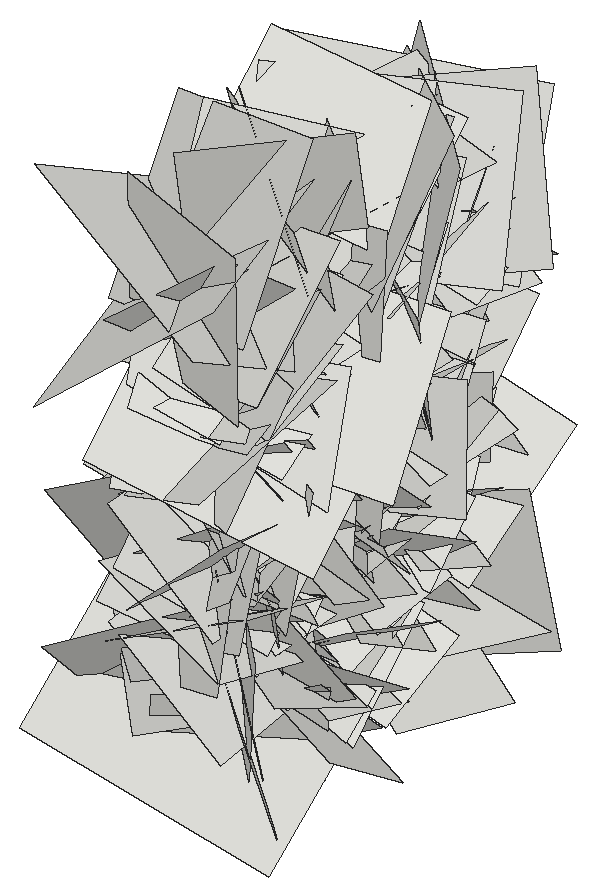
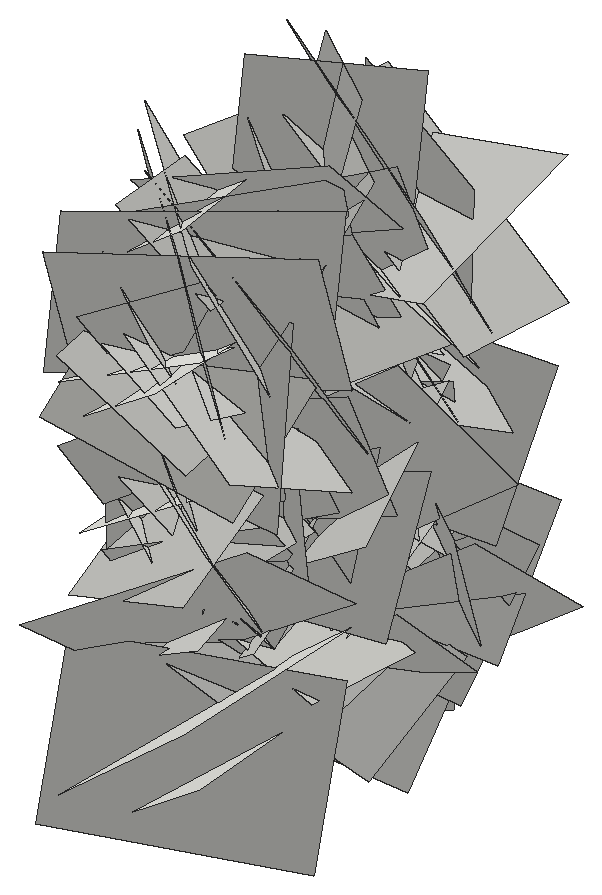
# SketchUp Ruby script. Lengths in inches.
U = 1.inch
M = Sketchup.active_model
def pt(a) = Geom::Point3d.new(a.map { |v| v * U })
def face(e, loops, mat)
  f = e.add_face(loops[0].map { |a| pt(a) })
  loops[1..].each { |l| e.add_face(l.map { |a| pt(a) }).erase! }
  f.material = f.back_material = mat if mat
  f
end
# faces: each face lists its corners as indices into pts; further lists are holes
def faces(e, pts, list, mat = nil) = list.each { |f| face(e, (f[0].is_a?(Array) ? f : [f]).map { |l| l.map { |i| pts[i] } }, mat) }
# xy, xz, yz: faces in a plane at the given z, y or x. An outline is a flat list of corners, or four numbers for a rectangle; further outlines are holes
def ring(l) = l.size == 4 ? [[l[0], l[1]], [l[2], l[1]], [l[2], l[3]], [l[0], l[3]]] : l.each_slice(2).to_a
def flat(e, list, mat, &to3) = list.each { |f| face(e, (f[0].is_a?(Array) ? f : [f]).map { |l| ring(l).map { |u, v| to3.(u, v) } }, mat) }
def xy(e, z, list, mat = nil) = flat(e, list, mat) { |x, y| [x, y, z] }
def xz(e, y, list, mat = nil) = flat(e, list, mat) { |x, z| [x, y, z] }
def yz(e, x, list, mat = nil) = flat(e, list, mat) { |y, z| [x, y, z] }
def lines(e, pts, list) = list.each { |a, b| e.add_line(pt(pts[a]), pt(pts[b])) }
# prism: a flat outline (further loops are holes) pulled along v
def prism(e, loops, v, mat = nil)
  f = face(e, loops, mat); d = Geom::Vector3d.new(v.map { |x| x * U })
  f.pushpull(f.normal.samedirection?(d) ? d.length : -d.length)
end
def box(e, o, s, mat = nil) = prism(e, [[o, [o[0] + s[0], o[1], o[2]], [o[0] + s[0], o[1] + s[1], o[2]], [o[0], o[1] + s[1], o[2]]]], [0, 0, s[2]], mat)
def at(x, y, z, deg = 0) = Geom::Transformation.translation(pt([x, y, z])) * Geom::Transformation.rotation(ORIGIN, Z_AXIS, deg.degrees)
def axes(o, x, y, z) = Geom::Transformation.new([*x, 0, *y, 0, *z, 0, *pt(o).to_a, 1])
def part(name) = M.definitions.add(name)
# library, detail: a bought-in or finely detailed component or shape, given as its bounding box
def library(name, o, s) = part(name).tap { |d| box(d.entities, o, s) }
def detail(e, o, s) = box(e.add_group.entities, o, s)
def put(e, d, t, mat = nil) = e.add_instance(d, t).tap { |i| i.material = mat if mat }
def group(e, t, mat = nil) = e.add_group.tap { |g| g.transformation = t; g.material = mat if mat }.entities
root = M.entities
c1 = part("Component\#6")
p = [[0.01,0,0],[0,3.24,4.54],[4.32,3.24,4.54],[4.33,0,0]]
faces(c1.entities,p,[[0,1,2,3]])
put(root,c1,axes([18.5,163.2,33.68],[-0.16473,-1.2102,0.57798],[-0.2383,0.59712,1.18983],[-1.40149,0.04071,-0.27024]))
put(root,c1,axes([18.5,157.9,37.93],[-0.24747,1.3445,0.30187],[0.11522,0.32319,-1.35538],[-1.4561,-0.20293,-0.15855]))
put(root,c1,axes([18.5,168.45,29.92],[-0.2904,-0.81126,-1.09363],[0.15157,-1.12651,0.79984],[-1.4354,0.04517,0.30571]))
put(root,c1,axes([18.5,159.18,36.25],[-0.04304,0.74935,1.15311],[-0.14712,1.14549,-0.74928],[-1.45028,-0.13844,0.04179]))
put(root,c1,axes([18.5,165.11,34.6875],[-0.03998,0.77126,1.05992],[-0.2457,1.03973,-0.76482],[-1.36759,-0.20934,0.10642]))
put(root,c1,axes([18.5,172.42,21.79],[-0.22827,-1.35966,0.24048],[0.1567,0.21929,1.3722],[-1.45519,0.2369,0.11004]))
put(root,c1,axes([18.5,158.06,26.05],[-0.19995,0.52409,1.06255],[-0.00833,1.07535,-0.5318],[-1.25583,-0.09057,-0.16565]))
put(root,c1,axes([18.5,166.62,31.96],[-0.21061,0.75098,-0.921],[0.02022,-0.93165,-0.76377],[-1.25951,-0.14053,0.14175]))
put(root,c1,axes([18.5,158.99,33.95],[-0.09747,0.08794,1.12692],[-0.17247,1.11783,-0.1005],[-1.18568,-0.16983,-0.07802]))
put(root,c1,axes([18.5,173.53,27.66],[-0.08068,-0.97468,-0.75893],[-0.01331,-0.75972,0.97695],[-1.30935,0.06778,0.03684]))
put(root,c1,axes([18.5,171.44,26.6],[0.03428,0.27698,-1.26013],[-0.06702,-1.25867,-0.27828],[-1.36598,0.0687,-0.01797]))
put(root,c1,axes([18.5,172.54,38.57],[0.12011,-0.4932,-1.18141],[-0.20578,-1.17893,0.47355],[-1.34134,0.1367,-0.17844]))
put(root,c1,axes([18.5,160.96,32.62],[-0.12215,0.75895,-0.88724],[-0.014,-0.89234,-0.7616],[-1.23753,-0.06482,0.09619]))
put(root,c1,axes([18.5,164.92,23.28],[-0.02573,-1.02703,-0.88101],[0.12942,-0.87922,1.02158],[-1.42847,-0.06116,0.10843]))
put(root,c1,axes([18.5,165.55,34.43],[0.04885,1.13911,0.54464],[-0.08516,0.54654,-1.13629],[-1.33566,0.00681,0.09237]))
put(root,c1,axes([18.5,166.97,25.06],[0.03339,-0.82276,-0.77538],[-0.30966,-0.75526,0.78954],[-1.15769,0.17829,-0.23355]))
put(root,c1,axes([18.5,159.8,34.2],[0.03301,0.77795,0.85676],[-0.24326,0.8442,-0.75821],[-1.20233,-0.14944,0.17692]))
put(root,c1,axes([18.5,169.63,32.59],[-0.01533,-0.4611,-1.03377],[-0.17767,-1.02158,0.45801],[-1.18663,0.15892,-0.05522]))
put(root,c1,axes([18.5,160.22,28.4],[-0.15479,0.80897,-0.76348],[0.02106,-0.76802,-0.81757],[-1.17891,-0.11994,0.08565]))
put(root,c1,axes([18.5,163.85,26.9],[-0.03329,1.04875,0.11229],[-0.24045,0.10299,-1.02538],[-1.09187,-0.05466,0.22238]))
put(root,c1,axes([18.5,168.84,39.14],[-0.0295,-0.69575,-0.73723],[-0.22295,-0.71749,0.68506],[-1.05113,0.17171,-0.12461]))
put(root,c1,axes([18.5,167.41,29.34],[0.20833,-0.42173,1.22713],[-0.0869,1.23461,0.43743],[-1.37269,-0.14217,0.15855]))
put(root,c1,axes([18.5,163.625,35.04],[-0.27654,-0.44632,0.88094],[0.09901,0.89592,0.48157],[-1.04211,0.20356,-0.18801]))
put(root,c1,axes([14.53,163.13,28.77],[-0.13219,-0.55975,0.33448],[-0.05965,0.34851,0.56225],[0.68862,-0.07726,0.11291]))
put(root,c1,axes([18.5,171.44,27.64],[-0.05126,-0.8571,0.56567],[-0.11133,0.56746,0.85083],[-1.08285,-0.01777,-0.11425]))
put(root,c1,axes([18.5,167.53,29.6],[-0.04916,0.6172,0.8297],[-0.08211,0.82613,-0.61887],[-1.09305,-0.08981,0.00917]))
put(root,c1,axes([18.5,170.89,20.28],[-0.12274,-1.02279,0.17958],[0.0333,0.17716,1.02926],[-1.10024,0.11946,0.01112]))
put(root,c1,axes([18.5,169.04,36.23],[0.04162,0.78981,-0.64322],[-0.24351,-0.62024,-0.77563],[-1.05189,0.17484,0.15411]))
put(root,c1,axes([14.53,163.1,21.29],[-0.03251,-0.459,0.52355],[-0.17075,0.51451,0.44164],[0.71801,0.10157,0.12873]))
put(root,c1,axes([18.5,158.58,28.72],[-0.17742,0.80309,0.64454],[0.10421,0.66248,-0.79991],[-1.08655,-0.0676,-0.18196]))
put(root,c1,axes([18.5,168.75,37.98],[0.06882,-0.53698,-1.12739],[0.1022,-1.12338,0.54063],[-1.31971,-0.115,-0.01692]))
put(root,c1,axes([18.5,166.67,25.47],[0.29316,-1.18227,0.54308],[-0.10516,0.53443,1.21398],[-1.37509,-0.29293,0.02294]))
put(root,c1,axes([14.53,169.1,21.1],[-0.05323,-0.42134,0.48328],[-0.06346,0.48572,0.41725],[0.67666,0.01241,0.07715]))
put(root,c1,axes([18.5,166.55,31.56],[-0.0814,0.41102,-0.8284],[-0.17089,-0.82447,-0.39413],[-0.96524,0.11131,0.13964]))
put(root,c1,axes([14.53,165.91,24.52],[0.03596,-0.58924,0.24858],[-0.15481,0.23521,0.57749],[0.65999,0.08727,0.12191]))
put(root,c1,axes([18.5,159.57,38.3125],[0.19748,1.37219,0.09956],[0.15298,0.08042,-1.37849],[-1.4503,0.19533,-0.13185]))
put(root,c1,axes([18.5,160.7,27.63],[0.09928,0.64406,-0.88513],[-0.13228,-0.87629,-0.65083],[-1.15276,0.15602,-0.00154]))
put(root,c1,axes([14.53,161.42,33.85],[-0.12931,-0.58697,0.4315],[-0.06321,0.44408,0.58723],[0.76963,-0.06214,0.12073]))
put(root,c1,axes([18.5,164.67,22.86],[0.07455,-1.03669,0.46758],[-0.01691,0.46753,1.03897],[-1.20537,-0.07068,0.01434]))
put(root,c1,axes([18.5,169.13,31.47],[-0.22896,-0.22184,-0.76377],[-0.12794,-0.77313,0.25869],[-0.83329,0.17965,0.17014]))
put(root,c1,axes([14.53,168.14,25.37],[-0.00005,-0.54267,0.44601],[-0.16088,0.43548,0.52984],[0.72699,0.09633,0.11728]))
put(root,c1,axes([14.53,167.47,38.84],[-0.19203,-0.25676,-0.78485],[-0.09527,-0.79261,0.28005],[0.87013,-0.14344,-0.14255]))
put(root,c1,axes([18.5,162.55,24.47],[-0.08094,0.6993,-0.63815],[-0.06519,-0.64254,-0.69674],[-1.00139,-0.01469,0.09694]))
put(root,c1,axes([18.5,168.37,37.02],[0.06582,-0.55881,-0.84289],[-0.17414,-0.83883,0.54402],[-1.05774,0.10333,-0.14201]))
put(root,c1,axes([14.53,168.24,29.62],[-0.00844,-0.1319,-0.59476],[-0.00779,-0.59475,0.132],[0.64572,-0.0089,-0.00618]))
put(root,c1,axes([14.53,163.79,31.02],[-0.0186,-0.39942,0.51021],[-0.04828,0.50989,0.39761],[0.68514,0.02509,0.04187]))
put(root,c1,axes([14.53,167.3,30.05],[-0.09755,-0.36279,0.79394],[-0.2327,0.7823,0.33203],[0.89554,0.16375,0.17276]))
put(root,c1,axes([14.53,166.74,28.03],[-0.20581,0.5378,0.53941],[0.0447,0.5634,-0.54654],[0.80617,0.10606,0.16802]))
put(root,c1,axes([14.53,165.16,26.22],[0.00662,-0.41647,0.48084],[-0.04981,0.47925,0.41571],[0.67246,0.0396,0.02606]))
put(root,c1,axes([18.5,162.15,25.43],[0.09766,0.84172,-0.54191],[-0.18116,-0.52299,-0.84139],[-1.04557,0.16923,0.09516]))
put(root,c1,axes([14.53,170.38,37.22],[-0.01844,-0.65259,0.06973],[-0.0154,0.07012,0.65262],[0.69551,-0.01575,0.0163]))
put(root,c1,axes([18.5,159.15,32.85],[0.28722,0.93511,0.86971],[0.00467,0.88838,-0.95656],[-1.35365,0.20148,0.18123]))
put(root,c1,axes([14.53,158.35,30.49],[-0.08461,0.81055,-0.03501],[-0.12527,-0.04642,-0.80528],[0.85081,0.07377,-0.12204]))
put(root,c1,axes([14.53,168.23,31.98],[-0.11552,-0.73847,0.10601],[0.00435,0.10653,0.74638],[0.79079,-0.10846,0.01138]))
put(root,c1,axes([14.53,162.33,29.83],[-0.22776,0.38392,-0.75072],[0.01782,-0.77261,-0.39993],[0.89361,0.11326,-0.18337]))
put(root,c1,axes([18.5,165.04,27.71],[0.04822,0.07219,0.94774],[-0.14201,0.93984,-0.06516],[-0.99746,-0.13032,0.05509]))
put(root,c1,axes([14.53,171.91,32.4],[0.07209,-0.36069,-0.54144],[-0.07785,-0.54516,0.35394],[0.6852,-0.024,0.09718]))
put(root,c1,axes([18.5,167.29,35.58],[-0.17595,-0.29467,-0.74084],[-0.05215,-0.7515,0.30993],[-0.84352,0.10793,0.13537]))
put(root,c1,axes([18.5,157.3125,32.29],[0.25179,1.05256,0.51222],[-0.06429,0.53303,-1.06718],[-1.23914,0.18623,0.15945]))
put(root,c1,axes([14.53,168.82,35.84],[0.04533,0.37689,0.51175],[-0.01637,0.51337,-0.3768],[0.67349,-0.01289,-0.04361]))
put(root,c1,axes([14.53,159.46,22.85],[-0.09982,-0.0635,0.89488],[-0.1784,0.88507,0.04509],[0.93408,0.16225,0.10424]))
put(root,c1,axes([14.53,160.06,22.6],[-0.02839,-0.24478,0.77995],[-0.15528,0.76918,0.23637],[0.85248,0.13195,0.06903]))
put(root,c1,axes([14.53,159.67,28.14],[-0.12868,0.67272,0.52517],[-0.08613,0.51893,-0.68352],[0.90053,0.14576,0.00967]))
put(root,c1,axes([14.53,158.39,26.84],[-0.02686,0.84806,0.10272],[-0.17857,0.09579,-0.83237],[0.88773,0.04493,-0.16432]))
put(root,c1,axes([14.53,169.17,27.35],[0.00515,-0.4485,-0.48712],[0.04455,-0.48594,0.44784],[0.70046,0.0342,-0.02491]))
put(root,c1,axes([18.5,161.79,25.53],[-0.01152,-0.82607,0.19056],[-0.15176,0.18963,0.81386],[-0.88572,-0.02175,-0.14193]))
put(root,c1,axes([18.5,164.2,31.01],[0.06613,-0.18181,-0.96198],[-0.02897,-0.96387,0.1804],[-1.03734,0.01533,-0.06637]))
put(root,c1,axes([14.53,169.92,30.86],[0.08798,0.07784,-0.70174],[-0.08853,-0.70052,-0.08758],[0.74315,-0.09267,0.07264]))
put(root,c1,axes([18.5,162.32,28.44],[-0.12821,-0.42216,-0.69512],[0.01339,-0.70366,0.42514],[-0.86197,0.05186,0.11]))
put(root,c1,axes([18.5,166.33,22.3],[0.05809,-0.87115,0.26873],[-0.09257,0.26296,0.87026],[-0.96191,-0.07791,-0.06752]))
put(root,c1,axes([18.5,171.77,39.47],[0.25632,-0.1505,-1.28885],[0.2021,-1.29268,0.18672],[-1.36053,-0.22038,-0.21508]))
put(root,c1,axes([14.53,167.69,34.89],[0.01272,-0.59445,-0.3878],[0.01652,-0.38754,0.59453],[0.75216,0.01856,-0.0065]))
put(root,c1,axes([14.53,168.18,25.35],[0.0356,-0.79141,-0.13903],[-0.13499,-0.14264,0.78117],[0.84098,0.01061,0.13127]))
put(root,c1,axes([18.5,163.85,33.45],[0.03445,-0.73428,-0.4148],[-0.17499,-0.41262,0.71747],[-0.87664,0.05351,-0.15952]))
put(root,c1,axes([18.5,158.45,30.92],[0.16236,0.46297,0.88251],[-0.09478,0.89566,-0.45434],[-1.05211,-0.00924,0.17712]))
put(root,c1,axes([18.5,166.53,31.68],[0.02185,0.89564,-0.0065],[-0.05171,-0.00537,-0.89456],[-0.948,0.02094,0.04865]))
put(root,c1,axes([18.5,171.21,38.93],[0.24063,-0.51313,-1.11059],[0.16085,-1.10901,0.54342],[-1.28679,-0.23458,-0.13976]))
put(root,c1,axes([14.53,171.89,34.33],[-0.10287,-0.74562,-0.1631],[0.15609,-0.17961,0.73351],[0.79385,-0.06131,-0.16536]))
put(root,c1,axes([18.5,162.43,26.35],[-0.02315,-0.70596,0.51236],[0.01203,0.51225,0.70629],[-0.92456,0.02434,-0.00364]))
put(root,c1,axes([18.5,162.61,28.57],[0.04222,-0.49534,0.62953],[-0.20196,0.60636,0.48917],[-0.82474,-0.17384,-0.08755]))
put(root,c1,axes([18.5,162.92,24.26],[-0.16568,0.16434,-0.80239],[0.1251,-0.80382,-0.18763],[-0.85913,-0.14874,0.12742]))
put(root,c1,axes([18.5,164.5,23.79],[-0.04443,0.667,0.37408],[-0.11412,0.36576,-0.66423],[-0.80255,-0.08894,0.07374]))
put(root,c1,axes([18.5,168.875,35.8],[-0.07444,0.7996,-0.0855],[-0.00091,-0.0859,-0.80263],[-0.85241,-0.06974,0.00832]))
put(root,c1,axes([14.53,164.96,33.58],[0.03363,-0.67551,-0.53197],[-0.14584,-0.52946,0.66412],[0.89967,-0.06058,0.12754]))
put(root,c1,axes([14.53,169.82,24.93],[0.00586,-0.68753,0.27068],[0.05817,0.27032,0.6855],[0.78107,-0.01497,-0.05308]))
put(root,c1,axes([18.5,164.8,26.41],[-0.06555,-0.88967,-0.10275],[0.1194,-0.1099,0.88381],[-0.94178,0.04799,0.1192]))
put(root,c1,axes([18.5,163.99,40.83],[-0.08038,0.23372,-0.81219],[0.10222,-0.80774,-0.24144],[-0.89001,-0.11388,0.04562]))
put(root,c1,axes([18.5,167.51,23.32],[0.04127,-0.8056,0.43064],[0.05085,0.43224,0.80425],[-0.96695,-0.01165,0.06068]))
put(root,c1,axes([18.5,164.95,29.96],[0.04265,0.57286,-0.52342],[-0.15347,-0.50938,-0.56862],[-0.80809,0.12697,0.08036]))
put(root,c1,axes([14.53,164.95,29.96],[-0.04265,0.57286,-0.52342],[0.15347,-0.50938,-0.56862],[0.80809,0.12697,0.08036]))
put(root,c1,axes([14.53,167.51,23.32],[-0.04127,-0.8056,0.43064],[-0.05085,0.43224,0.80425],[0.96695,-0.01165,0.06068]))
put(root,c1,axes([14.53,163.99,40.83],[0.08038,0.23372,-0.81219],[-0.10222,-0.80774,-0.24144],[0.89001,-0.11388,0.04562]))
put(root,c1,axes([14.53,164.8,26.41],[0.06555,-0.88967,-0.10275],[-0.1194,-0.1099,0.88381],[0.94178,0.04799,0.1192]))
put(root,c1,axes([18.5,169.82,24.93],[-0.00586,-0.68753,0.27068],[-0.05817,0.27032,0.6855],[-0.78107,-0.01497,-0.05308]))
put(root,c1,axes([18.5,164.96,33.58],[-0.03363,-0.67551,-0.53197],[0.14584,-0.52946,0.66412],[-0.89967,-0.06058,0.12754]))
put(root,c1,axes([14.53,168.875,35.8],[0.07444,0.7996,-0.0855],[0.00091,-0.0859,-0.80263],[0.85241,-0.06974,0.00832]))
put(root,c1,axes([14.53,164.5,23.79],[0.04443,0.667,0.37408],[0.11412,0.36576,-0.66423],[0.80255,-0.08894,0.07374]))
put(root,c1,axes([14.53,162.92,24.26],[0.16568,0.16434,-0.80239],[-0.1251,-0.80382,-0.18763],[0.85913,-0.14874,0.12742]))
put(root,c1,axes([14.53,162.61,28.57],[-0.04222,-0.49534,0.62953],[0.20196,0.60636,0.48917],[0.82474,-0.17384,-0.08755]))
put(root,c1,axes([14.53,162.43,26.35],[0.02315,-0.70596,0.51236],[-0.01203,0.51225,0.70629],[0.92456,0.02434,-0.00364]))
put(root,c1,axes([18.5,171.89,34.33],[0.10287,-0.74562,-0.1631],[-0.15609,-0.17961,0.73351],[-0.79385,-0.06131,-0.16536]))
put(root,c1,axes([14.53,171.21,38.93],[-0.24063,-0.51313,-1.11059],[-0.16085,-1.10901,0.54342],[1.28679,-0.23458,-0.13976]))
put(root,c1,axes([14.53,166.53,31.68],[-0.02185,0.89564,-0.0065],[0.05171,-0.00537,-0.89456],[0.948,0.02094,0.04865]))
put(root,c1,axes([14.53,158.45,30.92],[-0.16236,0.46297,0.88251],[0.09478,0.89566,-0.45434],[1.05211,-0.00924,0.17712]))
put(root,c1,axes([14.53,163.85,33.45],[-0.03445,-0.73428,-0.4148],[0.17499,-0.41262,0.71747],[0.87664,0.05351,-0.15952]))
put(root,c1,axes([18.5,168.18,25.35],[-0.0356,-0.79141,-0.13903],[0.13499,-0.14264,0.78117],[-0.84098,0.01061,0.13127]))
put(root,c1,axes([18.5,167.69,34.89],[-0.01272,-0.59445,-0.3878],[-0.01652,-0.38754,0.59453],[-0.75216,0.01856,-0.0065]))
put(root,c1,axes([14.53,171.77,39.47],[-0.25632,-0.1505,-1.28885],[-0.2021,-1.29268,0.18672],[1.36053,-0.22038,-0.21508]))
put(root,c1,axes([14.53,166.33,22.3],[-0.05809,-0.87115,0.26873],[0.09257,0.26296,0.87026],[0.96191,-0.07791,-0.06752]))
put(root,c1,axes([14.53,162.32,28.44],[0.12821,-0.42216,-0.69512],[-0.01339,-0.70366,0.42514],[0.86197,0.05186,0.11]))
put(root,c1,axes([18.5,169.92,30.86],[-0.08798,0.07784,-0.70174],[0.08853,-0.70052,-0.08758],[-0.74315,-0.09267,0.07264]))
put(root,c1,axes([14.53,164.2,31.01],[-0.06613,-0.18181,-0.96198],[0.02897,-0.96387,0.1804],[1.03734,0.01533,-0.06637]))
put(root,c1,axes([14.53,161.79,25.53],[0.01152,-0.82607,0.19056],[0.15176,0.18963,0.81386],[0.88572,-0.02175,-0.14193]))
put(root,c1,axes([18.5,169.17,27.35],[-0.00515,-0.4485,-0.48712],[-0.04455,-0.48594,0.44784],[-0.70046,0.0342,-0.02491]))
put(root,c1,axes([18.5,158.39,26.84],[0.02686,0.84806,0.10272],[0.17857,0.09579,-0.83237],[-0.88773,0.04493,-0.16432]))
put(root,c1,axes([18.5,159.67,28.14],[0.12868,0.67272,0.52517],[0.08613,0.51893,-0.68352],[-0.90053,0.14576,0.00967]))
put(root,c1,axes([18.5,160.06,22.6],[0.02839,-0.24478,0.77995],[0.15528,0.76918,0.23637],[-0.85248,0.13195,0.06903]))
put(root,c1,axes([18.5,159.46,22.85],[0.09982,-0.0635,0.89488],[0.1784,0.88507,0.04509],[-0.93408,0.16225,0.10424]))
put(root,c1,axes([18.5,168.82,35.84],[-0.04533,0.37689,0.51175],[0.01637,0.51337,-0.3768],[-0.67349,-0.01289,-0.04361]))
put(root,c1,axes([14.53,157.3125,32.29],[-0.25179,1.05256,0.51222],[0.06429,0.53303,-1.06718],[1.23914,0.18623,0.15945]))
put(root,c1,axes([14.53,167.29,35.58],[0.17595,-0.29467,-0.74084],[0.05215,-0.7515,0.30993],[0.84352,0.10793,0.13537]))
put(root,c1,axes([18.5,171.91,32.4],[-0.07209,-0.36069,-0.54144],[0.07785,-0.54516,0.35394],[-0.6852,-0.024,0.09718]))
put(root,c1,axes([14.53,165.04,27.71],[-0.04822,0.07219,0.94774],[0.14201,0.93984,-0.06516],[0.99746,-0.13032,0.05509]))
put(root,c1,axes([18.5,162.33,29.83],[0.22776,0.38392,-0.75072],[-0.01782,-0.77261,-0.39993],[-0.89361,0.11326,-0.18337]))
put(root,c1,axes([18.5,168.23,31.98],[0.11552,-0.73847,0.10601],[-0.00435,0.10653,0.74638],[-0.79079,-0.10846,0.01138]))
put(root,c1,axes([18.5,158.35,30.49],[0.08461,0.81055,-0.03501],[0.12527,-0.04642,-0.80528],[-0.85081,0.07377,-0.12204]))
put(root,c1,axes([14.53,159.15,32.85],[-0.28722,0.93511,0.86971],[-0.00467,0.88838,-0.95656],[1.35365,0.20148,0.18123]))
put(root,c1,axes([18.5,170.38,37.22],[0.01844,-0.65259,0.06973],[0.0154,0.07012,0.65262],[-0.69551,-0.01575,0.0163]))
put(root,c1,axes([14.53,162.15,25.43],[-0.09766,0.84172,-0.54191],[0.18116,-0.52299,-0.84139],[1.04557,0.16923,0.09516]))
put(root,c1,axes([18.5,165.16,26.22],[-0.00662,-0.41647,0.48084],[0.04981,0.47925,0.41571],[-0.67246,0.0396,0.02606]))
put(root,c1,axes([18.5,166.74,28.03],[0.20581,0.5378,0.53941],[-0.0447,0.5634,-0.54654],[-0.80617,0.10606,0.16802]))
put(root,c1,axes([18.5,167.3,30.05],[0.09755,-0.36279,0.79394],[0.2327,0.7823,0.33203],[-0.89554,0.16375,0.17276]))
put(root,c1,axes([18.5,163.79,31.02],[0.0186,-0.39942,0.51021],[0.04828,0.50989,0.39761],[-0.68514,0.02509,0.04187]))
